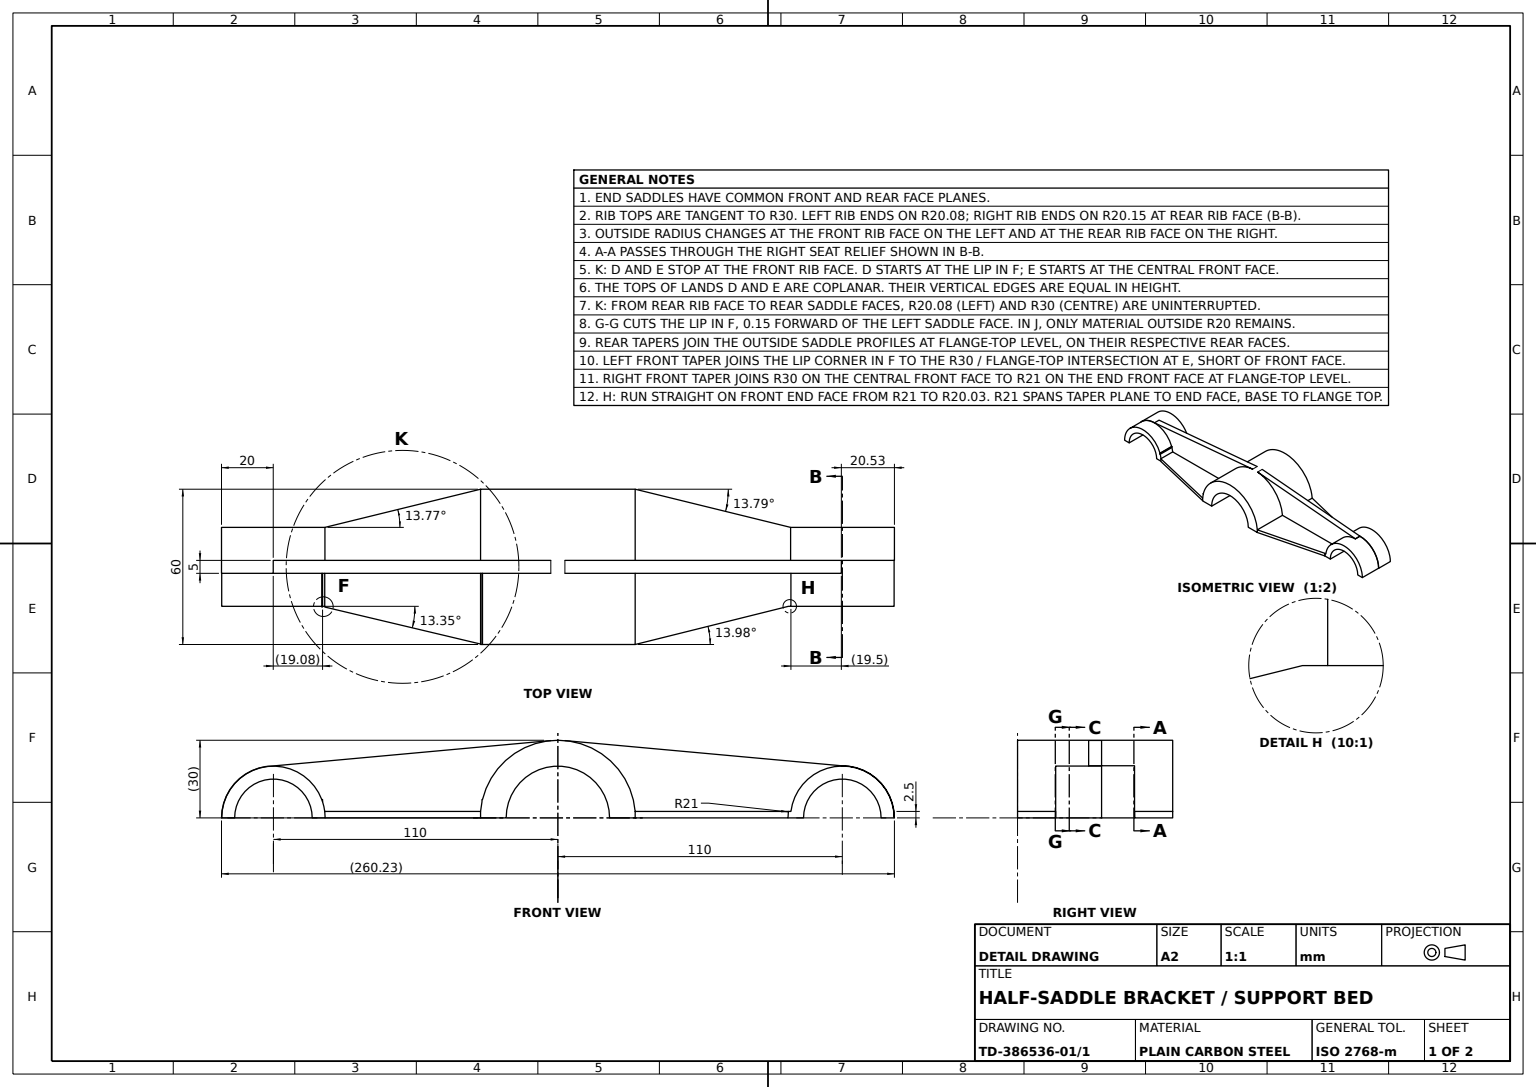
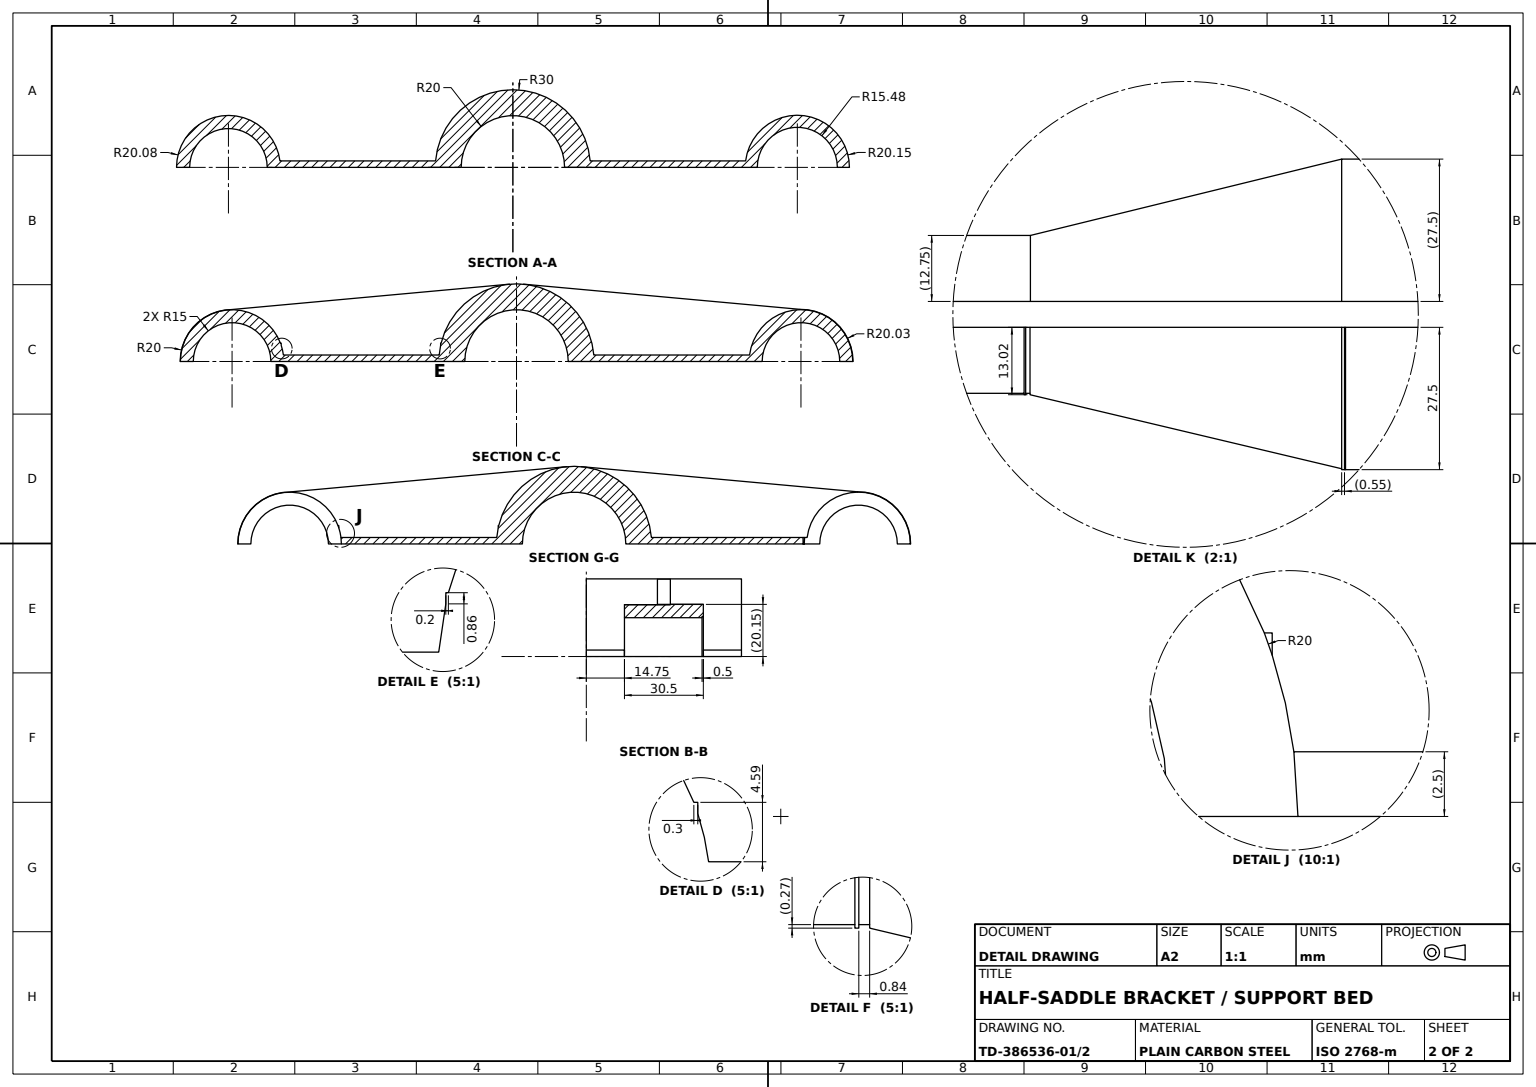
ISO-10303-21;
HEADER;
FILE_DESCRIPTION((''),'2;1');
FILE_NAME('','',(''),(''),'','','');
FILE_SCHEMA(('AUTOMOTIVE_DESIGN'));
ENDSEC;
DATA;
#1=APPLICATION_CONTEXT('');
#2=PRODUCT_CONTEXT('',#1,'mechanical');
#3=PRODUCT('','','',(#2));
#4=PRODUCT_DEFINITION_FORMATION('','',#3);
#5=PRODUCT_DEFINITION_CONTEXT('',#1,'design');
#6=PRODUCT_DEFINITION('','',#4,#5);
#7=PRODUCT_DEFINITION_SHAPE('','',#6);
#8=(LENGTH_UNIT()NAMED_UNIT(*)SI_UNIT(.MILLI.,.METRE.));
#9=(NAMED_UNIT(*)PLANE_ANGLE_UNIT()SI_UNIT($,.RADIAN.));
#10=(NAMED_UNIT(*)SI_UNIT($,.STERADIAN.)SOLID_ANGLE_UNIT());
#11=UNCERTAINTY_MEASURE_WITH_UNIT(LENGTH_MEASURE(1.E-05),#8,'distance_accuracy_value','');
#12=(GEOMETRIC_REPRESENTATION_CONTEXT(3)GLOBAL_UNCERTAINTY_ASSIGNED_CONTEXT((#11))GLOBAL_UNIT_ASSIGNED_CONTEXT((#8,#9,#10))REPRESENTATION_CONTEXT('',''));
#13=CARTESIAN_POINT('',(109.62431,20.147505,70.));
#14=VERTEX_POINT('',#13);
#15=CARTESIAN_POINT('',(109.62431,20.027015,70.));
#16=VERTEX_POINT('',#15);
#17=CARTESIAN_POINT('',(109.62431,0.,70.));
#18=DIRECTION('',(0.,-1.,0.));
#19=VECTOR('',#18,1000.);
#20=LINE('',#17,#19);
#21=EDGE_CURVE('',#14,#16,#20,.T.);
#22=ORIENTED_EDGE('',*,*,#21,.F.);
#23=CARTESIAN_POINT('',(109.62431,20.147505,75.));
#24=VERTEX_POINT('',#23);
#25=DIRECTION('',(0.,0.,1.));
#26=VECTOR('',#25,1000.);
#27=LINE('',#13,#26);
#28=EDGE_CURVE('',#14,#24,#27,.T.);
#29=ORIENTED_EDGE('',*,*,#28,.T.);
#30=CARTESIAN_POINT('',(109.62431,20.027015,75.));
#31=VERTEX_POINT('',#30);
#32=CARTESIAN_POINT('',(109.62431,0.,75.));
#33=LINE('',#32,#19);
#34=EDGE_CURVE('',#24,#31,#33,.T.);
#35=ORIENTED_EDGE('',*,*,#34,.T.);
#36=DIRECTION('',(0.,0.,-1.));
#37=VECTOR('',#36,1000.);
#38=LINE('',#30,#37);
#39=EDGE_CURVE('',#31,#16,#38,.T.);
#40=ORIENTED_EDGE('',*,*,#39,.T.);
#41=EDGE_LOOP('',(#22,#29,#35,#40));
#42=FACE_OUTER_BOUND('',#41,.T.);
#43=DIRECTION('',(-1.,0.,0.));
#44=AXIS2_PLACEMENT_3D('',#17,#43,#25);
#45=PLANE('',#44);
#46=ADVANCED_FACE('',(#42),#45,.F.);
#47=CARTESIAN_POINT('',(-89.923483,0.,57.211703));
#48=VERTEX_POINT('',#47);
#49=CARTESIAN_POINT('',(-29.895652,0.,42.5));
#50=VERTEX_POINT('',#49);
#51=CARTESIAN_POINT('',(-90.079745,0.,57.25));
#52=DIRECTION('',(0.97125614,0.,-0.238036784));
#53=VECTOR('',#52,1000.);
#54=LINE('',#51,#53);
#55=EDGE_CURVE('',#48,#50,#54,.T.);
#56=ORIENTED_EDGE('',*,*,#55,.F.);
#57=CARTESIAN_POINT('',(-90.079745,2.5,57.25));
#58=VERTEX_POINT('',#57);
#59=CARTESIAN_POINT('',(-89.923483,0.836045,57.211703));
#60=CARTESIAN_POINT('',(-89.975638,1.670462,57.224485));
#61=(BOUNDED_CURVE()B_SPLINE_CURVE(3,(#47,#59,#60,#57),.UNSPECIFIED.,.F.,.T.)B_SPLINE_CURVE_WITH_KNOTS((4,4),(0.,0.12484767),.UNSPECIFIED.)CURVE()GEOMETRIC_REPRESENTATION_ITEM()RATIONAL_B_SPLINE_CURVE((1.,0.99870151,0.99870151,1.))REPRESENTATION_ITEM(''));
#62=EDGE_CURVE('',#48,#58,#61,.T.);
#63=ORIENTED_EDGE('',*,*,#62,.T.);
#64=CARTESIAN_POINT('',(-29.895652,2.5,42.5));
#65=VERTEX_POINT('',#64);
#66=CARTESIAN_POINT('',(-1.693933,2.5,35.588284));
#67=DIRECTION('',(-0.97125614,0.,0.238036784));
#68=VECTOR('',#67,1000.);
#69=LINE('',#66,#68);
#70=EDGE_CURVE('',#65,#58,#69,.T.);
#71=ORIENTED_EDGE('',*,*,#70,.F.);
#72=CARTESIAN_POINT('',(-29.895652,68.5,42.5));
#73=LINE('',#72,#19);
#74=EDGE_CURVE('',#65,#50,#73,.T.);
#75=ORIENTED_EDGE('',*,*,#74,.T.);
#76=EDGE_LOOP('',(#56,#63,#71,#75));
#77=FACE_OUTER_BOUND('',#76,.T.);
#78=CARTESIAN_POINT('',(-90.079745,68.5,57.25));
#79=DIRECTION('',(-0.238036784,0.,-0.97125614));
#80=AXIS2_PLACEMENT_3D('',#78,#79,#67);
#81=PLANE('',#80);
#82=ADVANCED_FACE('',(#77),#81,.T.);
#83=CARTESIAN_POINT('',(29.895652,2.5,42.5));
#84=VERTEX_POINT('',#83);
#85=CARTESIAN_POINT('',(29.895652,2.5,70.));
#86=VERTEX_POINT('',#85);
#87=LINE('',#83,#26);
#88=EDGE_CURVE('',#84,#86,#87,.T.);
#89=ORIENTED_EDGE('',*,*,#88,.F.);
#90=CARTESIAN_POINT('',(0.,0.,42.5));
#91=AXIS2_PLACEMENT_3D('',#90,#36,#43);
#92=CIRCLE('',#91,30.);
#93=EDGE_CURVE('',#65,#84,#92,.T.);
#94=ORIENTED_EDGE('',*,*,#93,.F.);
#95=CARTESIAN_POINT('',(-29.895652,2.5,70.));
#96=VERTEX_POINT('',#95);
#97=LINE('',#64,#26);
#98=EDGE_CURVE('',#65,#96,#97,.T.);
#99=ORIENTED_EDGE('',*,*,#98,.T.);
#100=CARTESIAN_POINT('',(-2.727273,29.875776,70.));
#101=VERTEX_POINT('',#100);
#102=CARTESIAN_POINT('',(0.,0.,70.));
#103=AXIS2_PLACEMENT_3D('',#102,#25,#43);
#104=CIRCLE('',#103,30.);
#105=EDGE_CURVE('',#101,#96,#104,.T.);
#106=ORIENTED_EDGE('',*,*,#105,.F.);
#107=CARTESIAN_POINT('',(-2.727273,29.875776,75.));
#108=VERTEX_POINT('',#107);
#109=LINE('',#107,#37);
#110=EDGE_CURVE('',#108,#101,#109,.T.);
#111=ORIENTED_EDGE('',*,*,#110,.F.);
#112=CARTESIAN_POINT('',(-29.149589,7.092351,75.));
#113=VERTEX_POINT('',#112);
#114=CARTESIAN_POINT('',(0.,0.,75.));
#115=DIRECTION('',(1.,0.,0.));
#116=AXIS2_PLACEMENT_3D('',#114,#25,#115);
#117=CIRCLE('',#116,30.);
#118=EDGE_CURVE('',#108,#113,#117,.T.);
#119=ORIENTED_EDGE('',*,*,#118,.T.);
#120=CARTESIAN_POINT('',(-29.149589,7.092351,102.5));
#121=VERTEX_POINT('',#120);
#122=LINE('',#120,#37);
#123=EDGE_CURVE('',#121,#113,#122,.T.);
#124=ORIENTED_EDGE('',*,*,#123,.F.);
#125=CARTESIAN_POINT('',(29.895652,2.5,102.5));
#126=VERTEX_POINT('',#125);
#127=CARTESIAN_POINT('',(0.,0.,102.5));
#128=AXIS2_PLACEMENT_3D('',#127,#25,#115);
#129=CIRCLE('',#128,30.);
#130=EDGE_CURVE('',#126,#121,#129,.T.);
#131=ORIENTED_EDGE('',*,*,#130,.F.);
#132=CARTESIAN_POINT('',(29.895652,2.5,75.));
#133=VERTEX_POINT('',#132);
#134=LINE('',#125,#37);
#135=EDGE_CURVE('',#126,#133,#134,.T.);
#136=ORIENTED_EDGE('',*,*,#135,.T.);
#137=CARTESIAN_POINT('',(2.718944,29.876535,75.));
#138=VERTEX_POINT('',#137);
#139=EDGE_CURVE('',#133,#138,#117,.T.);
#140=ORIENTED_EDGE('',*,*,#139,.T.);
#141=CARTESIAN_POINT('',(2.718944,29.876535,70.));
#142=VERTEX_POINT('',#141);
#143=LINE('',#141,#26);
#144=EDGE_CURVE('',#142,#138,#143,.T.);
#145=ORIENTED_EDGE('',*,*,#144,.F.);
#146=EDGE_CURVE('',#86,#142,#104,.T.);
#147=ORIENTED_EDGE('',*,*,#146,.F.);
#148=EDGE_LOOP('',(#89,#94,#99,#106,#111,#119,#124,#131,#136,#140,#145,#147));
#149=FACE_OUTER_BOUND('',#148,.T.);
#150=CARTESIAN_POINT('',(0.,0.,20.));
#151=AXIS2_PLACEMENT_3D('',#150,#36,#43);
#152=CYLINDRICAL_SURFACE('',#151,30.);
#153=ADVANCED_FACE('',(#149),#152,.T.);
#154=CARTESIAN_POINT('',(-90.156865,2.5,88.021244));
#155=VERTEX_POINT('',#154);
#156=CARTESIAN_POINT('',(-90.,0.,88.058473));
#157=VERTEX_POINT('',#156);
#158=CARTESIAN_POINT('',(-90.052357,1.670491,88.046047));
#159=CARTESIAN_POINT('',(-90.,0.836066,88.058473));
#160=(BOUNDED_CURVE()B_SPLINE_CURVE(3,(#154,#158,#159,#156),.UNSPECIFIED.,.F.,.F.)B_SPLINE_CURVE_WITH_KNOTS((4,4),(6.157857476,6.283185307),.UNSPECIFIED.)CURVE()GEOMETRIC_REPRESENTATION_ITEM()RATIONAL_B_SPLINE_CURVE((1.,0.998691506,0.998691506,1.))REPRESENTATION_ITEM(''));
#161=EDGE_CURVE('',#155,#157,#160,.T.);
#162=ORIENTED_EDGE('',*,*,#161,.F.);
#163=CARTESIAN_POINT('',(-90.156865,2.5,87.75));
#164=VERTEX_POINT('',#163);
#165=CARTESIAN_POINT('',(-90.156865,2.5,102.5));
#166=LINE('',#165,#37);
#167=EDGE_CURVE('',#155,#164,#166,.T.);
#168=ORIENTED_EDGE('',*,*,#167,.T.);
#169=CARTESIAN_POINT('',(-90.,0.,87.75));
#170=VERTEX_POINT('',#169);
#171=CARTESIAN_POINT('',(-110.,0.,87.75));
#172=AXIS2_PLACEMENT_3D('',#171,#25,#115);
#173=CIRCLE('',#172,20.);
#174=EDGE_CURVE('',#170,#164,#173,.T.);
#175=ORIENTED_EDGE('',*,*,#174,.F.);
#176=LINE('',#169,#26);
#177=EDGE_CURVE('',#170,#157,#176,.T.);
#178=ORIENTED_EDGE('',*,*,#177,.T.);
#179=EDGE_LOOP('',(#162,#168,#175,#178));
#180=FACE_OUTER_BOUND('',#179,.T.);
#181=CYLINDRICAL_SURFACE('',#172,20.);
#182=ADVANCED_FACE('',(#180),#181,.F.);
#183=CARTESIAN_POINT('',(-91.299771,7.092351,75.));
#184=VERTEX_POINT('',#183);
#185=CARTESIAN_POINT('',(-130.,0.,75.));
#186=VERTEX_POINT('',#185);
#187=CARTESIAN_POINT('',(-110.,0.,75.));
#188=AXIS2_PLACEMENT_3D('',#187,#25,#43);
#189=CIRCLE('',#188,20.);
#190=EDGE_CURVE('',#184,#186,#189,.T.);
#191=ORIENTED_EDGE('',*,*,#190,.T.);
#192=CARTESIAN_POINT('',(-130.,0.,87.75));
#193=VERTEX_POINT('',#192);
#194=CARTESIAN_POINT('',(-130.,0.,102.5));
#195=LINE('',#194,#26);
#196=EDGE_CURVE('',#186,#193,#195,.T.);
#197=ORIENTED_EDGE('',*,*,#196,.T.);
#198=CARTESIAN_POINT('',(-91.299771,7.092351,87.75));
#199=VERTEX_POINT('',#198);
#200=EDGE_CURVE('',#199,#193,#173,.T.);
#201=ORIENTED_EDGE('',*,*,#200,.F.);
#202=CARTESIAN_POINT('',(-91.299771,7.092351,102.5));
#203=LINE('',#202,#37);
#204=EDGE_CURVE('',#199,#184,#203,.T.);
#205=ORIENTED_EDGE('',*,*,#204,.T.);
#206=EDGE_LOOP('',(#191,#197,#201,#205));
#207=FACE_OUTER_BOUND('',#206,.T.);
#208=CARTESIAN_POINT('',(-110.,0.,102.5));
#209=AXIS2_PLACEMENT_3D('',#208,#36,#43);
#210=CYLINDRICAL_SURFACE('',#209,20.);
#211=ADVANCED_FACE('',(#207),#210,.T.);
#212=CARTESIAN_POINT('',(29.895652,0.,102.5));
#213=VERTEX_POINT('',#212);
#214=CARTESIAN_POINT('',(29.895652,-99.5,102.5));
#215=DIRECTION('',(0.,1.,0.));
#216=VECTOR('',#215,1000.);
#217=LINE('',#214,#216);
#218=EDGE_CURVE('',#213,#126,#217,.T.);
#219=ORIENTED_EDGE('',*,*,#218,.F.);
#220=CARTESIAN_POINT('',(89.,0.,87.787175));
#221=VERTEX_POINT('',#220);
#222=DIRECTION('',(-0.970386397,0.,0.241557946));
#223=VECTOR('',#222,1000.);
#224=LINE('',#212,#223);
#225=EDGE_CURVE('',#221,#213,#224,.T.);
#226=ORIENTED_EDGE('',*,*,#225,.F.);
#227=CARTESIAN_POINT('',(89.149341,2.5,87.75));
#228=VERTEX_POINT('',#227);
#229=CARTESIAN_POINT('',(89.049839,1.670133,87.774769));
#230=CARTESIAN_POINT('',(89.,0.83581,87.787175));
#231=(BOUNDED_CURVE()B_SPLINE_CURVE(3,(#227,#229,#230,#220),.UNSPECIFIED.,.F.,.F.)B_SPLINE_CURVE_WITH_KNOTS((4,4),(3.022262029,3.141592654),.UNSPECIFIED.)CURVE()GEOMETRIC_REPRESENTATION_ITEM()RATIONAL_B_SPLINE_CURVE((1.,0.998813702,0.998813702,1.))REPRESENTATION_ITEM(''));
#232=EDGE_CURVE('',#228,#221,#231,.T.);
#233=ORIENTED_EDGE('',*,*,#232,.F.);
#234=CARTESIAN_POINT('',(1.744419,2.5,109.507677));
#235=DIRECTION('',(0.970386397,0.,-0.241557946));
#236=VECTOR('',#235,1000.);
#237=LINE('',#234,#236);
#238=EDGE_CURVE('',#126,#228,#237,.T.);
#239=ORIENTED_EDGE('',*,*,#238,.F.);
#240=EDGE_LOOP('',(#219,#226,#233,#239));
#241=FACE_OUTER_BOUND('',#240,.T.);
#242=DIRECTION('',(0.241557946,0.,0.970386397));
#243=AXIS2_PLACEMENT_3D('',#214,#242,#235);
#244=PLANE('',#243);
#245=ADVANCED_FACE('',(#241),#244,.T.);
#246=CARTESIAN_POINT('',(-110.074279,20.07638,70.));
#247=VERTEX_POINT('',#246);
#248=CARTESIAN_POINT('',(-90.079745,2.5,70.));
#249=VERTEX_POINT('',#248);
#250=CARTESIAN_POINT('',(-110.,0.,70.));
#251=AXIS2_PLACEMENT_3D('',#250,#36,#43);
#252=CIRCLE('',#251,20.076517);
#253=EDGE_CURVE('',#247,#249,#252,.T.);
#254=ORIENTED_EDGE('',*,*,#253,.F.);
#255=DIRECTION('',(-0.995859195,-0.090909091,0.));
#256=VECTOR('',#255,1000.);
#257=LINE('',#100,#256);
#258=EDGE_CURVE('',#101,#247,#257,.T.);
#259=ORIENTED_EDGE('',*,*,#258,.F.);
#260=ORIENTED_EDGE('',*,*,#105,.T.);
#261=CARTESIAN_POINT('',(0.,2.5,70.));
#262=VECTOR('',#43,1000.);
#263=LINE('',#261,#262);
#264=EDGE_CURVE('',#96,#249,#263,.T.);
#265=ORIENTED_EDGE('',*,*,#264,.T.);
#266=EDGE_LOOP('',(#254,#259,#260,#265));
#267=FACE_OUTER_BOUND('',#266,.T.);
#268=AXIS2_PLACEMENT_3D('',#102,#36,#43);
#269=PLANE('',#268);
#270=ADVANCED_FACE('',(#267),#269,.T.);
#271=CARTESIAN_POINT('',(-90.156865,2.5,75.));
#272=VERTEX_POINT('',#271);
#273=EDGE_CURVE('',#164,#272,#166,.T.);
#274=ORIENTED_EDGE('',*,*,#273,.T.);
#275=CARTESIAN_POINT('',(-90.995037,6.229877,75.));
#276=VERTEX_POINT('',#275);
#277=EDGE_CURVE('',#272,#276,#189,.T.);
#278=ORIENTED_EDGE('',*,*,#277,.T.);
#279=CARTESIAN_POINT('',(-90.995037,6.229877,87.75));
#280=VERTEX_POINT('',#279);
#281=CARTESIAN_POINT('',(-90.995037,6.229877,102.5));
#282=LINE('',#281,#37);
#283=EDGE_CURVE('',#280,#276,#282,.T.);
#284=ORIENTED_EDGE('',*,*,#283,.F.);
#285=EDGE_CURVE('',#164,#280,#173,.T.);
#286=ORIENTED_EDGE('',*,*,#285,.F.);
#287=EDGE_LOOP('',(#274,#278,#284,#286));
#288=FACE_OUTER_BOUND('',#287,.T.);
#289=ADVANCED_FACE('',(#288),#210,.T.);
#290=CARTESIAN_POINT('',(-90.995037,7.092351,75.));
#291=VERTEX_POINT('',#290);
#292=CARTESIAN_POINT('',(-90.995037,0.,75.));
#293=LINE('',#292,#19);
#294=EDGE_CURVE('',#291,#276,#293,.T.);
#295=ORIENTED_EDGE('',*,*,#294,.F.);
#296=CARTESIAN_POINT('',(-90.995037,7.092351,88.021244));
#297=VERTEX_POINT('',#296);
#298=CARTESIAN_POINT('',(-90.995037,7.092351,102.5));
#299=LINE('',#298,#37);
#300=EDGE_CURVE('',#297,#291,#299,.T.);
#301=ORIENTED_EDGE('',*,*,#300,.F.);
#302=CARTESIAN_POINT('',(-90.995037,6.229877,88.021244));
#303=VERTEX_POINT('',#302);
#304=CARTESIAN_POINT('',(-90.995037,-57.229877,88.021244));
#305=LINE('',#304,#216);
#306=EDGE_CURVE('',#303,#297,#305,.T.);
#307=ORIENTED_EDGE('',*,*,#306,.F.);
#308=EDGE_CURVE('',#303,#280,#282,.T.);
#309=ORIENTED_EDGE('',*,*,#308,.T.);
#310=ORIENTED_EDGE('',*,*,#283,.T.);
#311=EDGE_LOOP('',(#295,#301,#307,#309,#310));
#312=FACE_OUTER_BOUND('',#311,.T.);
#313=CARTESIAN_POINT('',(-90.995037,-57.229877,75.));
#314=AXIS2_PLACEMENT_3D('',#313,#115,#36);
#315=PLANE('',#314);
#316=ADVANCED_FACE('',(#312),#315,.T.);
#317=CARTESIAN_POINT('',(125.480421,0.,57.75));
#318=VERTEX_POINT('',#317);
#319=CARTESIAN_POINT('',(94.519579,0.,57.75));
#320=VERTEX_POINT('',#319);
#321=CARTESIAN_POINT('',(110.,0.,57.75));
#322=AXIS2_PLACEMENT_3D('',#321,#25,#115);
#323=CIRCLE('',#322,15.480421);
#324=EDGE_CURVE('',#318,#320,#323,.T.);
#325=ORIENTED_EDGE('',*,*,#324,.T.);
#326=CARTESIAN_POINT('',(94.519579,0.,57.25));
#327=VERTEX_POINT('',#326);
#328=CARTESIAN_POINT('',(94.519579,0.,47.75));
#329=LINE('',#328,#37);
#330=EDGE_CURVE('',#320,#327,#329,.T.);
#331=ORIENTED_EDGE('',*,*,#330,.T.);
#332=CARTESIAN_POINT('',(125.480421,0.,57.25));
#333=VERTEX_POINT('',#332);
#334=CARTESIAN_POINT('',(110.,0.,57.25));
#335=AXIS2_PLACEMENT_3D('',#334,#36,#43);
#336=CIRCLE('',#335,15.480421);
#337=EDGE_CURVE('',#327,#333,#336,.T.);
#338=ORIENTED_EDGE('',*,*,#337,.T.);
#339=CARTESIAN_POINT('',(125.480421,0.,47.75));
#340=LINE('',#339,#26);
#341=EDGE_CURVE('',#333,#318,#340,.T.);
#342=ORIENTED_EDGE('',*,*,#341,.T.);
#343=EDGE_LOOP('',(#325,#331,#338,#342));
#344=FACE_OUTER_BOUND('',#343,.T.);
#345=CARTESIAN_POINT('',(110.,0.,47.75));
#346=AXIS2_PLACEMENT_3D('',#345,#25,#115);
#347=CYLINDRICAL_SURFACE('',#346,15.480421);
#348=ADVANCED_FACE('',(#344),#347,.F.);
#349=CARTESIAN_POINT('',(-91.299771,7.092351,88.021244));
#350=VERTEX_POINT('',#349);
#351=EDGE_CURVE('',#350,#199,#203,.T.);
#352=ORIENTED_EDGE('',*,*,#351,.T.);
#353=EDGE_CURVE('',#280,#199,#173,.T.);
#354=ORIENTED_EDGE('',*,*,#353,.F.);
#355=ORIENTED_EDGE('',*,*,#308,.F.);
#356=CARTESIAN_POINT('',(-110.,0.,88.021244));
#357=AXIS2_PLACEMENT_3D('',#356,#25,#43);
#358=CIRCLE('',#357,20.);
#359=EDGE_CURVE('',#303,#350,#358,.T.);
#360=ORIENTED_EDGE('',*,*,#359,.T.);
#361=EDGE_LOOP('',(#352,#354,#355,#360));
#362=FACE_OUTER_BOUND('',#361,.T.);
#363=ADVANCED_FACE('',(#362),#181,.F.);
#364=CARTESIAN_POINT('',(130.151008,0.,70.));
#365=VERTEX_POINT('',#364);
#366=CARTESIAN_POINT('',(110.,0.,70.));
#367=AXIS2_PLACEMENT_3D('',#366,#36,#43);
#368=CIRCLE('',#367,20.151008);
#369=EDGE_CURVE('',#14,#365,#368,.T.);
#370=ORIENTED_EDGE('',*,*,#369,.T.);
#371=CARTESIAN_POINT('',(130.151008,0.,57.25));
#372=VERTEX_POINT('',#371);
#373=CARTESIAN_POINT('',(130.151008,0.,42.5));
#374=LINE('',#373,#37);
#375=EDGE_CURVE('',#365,#372,#374,.T.);
#376=ORIENTED_EDGE('',*,*,#375,.T.);
#377=CARTESIAN_POINT('',(90.004673,2.5,57.25));
#378=VERTEX_POINT('',#377);
#379=CIRCLE('',#335,20.151008);
#380=EDGE_CURVE('',#378,#372,#379,.T.);
#381=ORIENTED_EDGE('',*,*,#380,.F.);
#382=CARTESIAN_POINT('',(90.004673,2.5,70.));
#383=VERTEX_POINT('',#382);
#384=CARTESIAN_POINT('',(90.004673,2.5,42.5));
#385=LINE('',#384,#26);
#386=EDGE_CURVE('',#378,#383,#385,.T.);
#387=ORIENTED_EDGE('',*,*,#386,.T.);
#388=AXIS2_PLACEMENT_3D('',#366,#36,#115);
#389=CIRCLE('',#388,20.151008);
#390=EDGE_CURVE('',#383,#14,#389,.T.);
#391=ORIENTED_EDGE('',*,*,#390,.T.);
#392=EDGE_LOOP('',(#370,#376,#381,#387,#391));
#393=FACE_OUTER_BOUND('',#392,.T.);
#394=CARTESIAN_POINT('',(110.,0.,42.5));
#395=AXIS2_PLACEMENT_3D('',#394,#25,#115);
#396=CYLINDRICAL_SURFACE('',#395,20.151008);
#397=ADVANCED_FACE('',(#393),#396,.T.);
#398=CARTESIAN_POINT('',(20.,0.,102.5));
#399=VERTEX_POINT('',#398);
#400=CARTESIAN_POINT('',(-20.,0.,102.5));
#401=VERTEX_POINT('',#400);
#402=CIRCLE('',#128,20.);
#403=EDGE_CURVE('',#399,#401,#402,.T.);
#404=ORIENTED_EDGE('',*,*,#403,.T.);
#405=CARTESIAN_POINT('',(-20.,0.,42.5));
#406=VERTEX_POINT('',#405);
#407=CARTESIAN_POINT('',(-20.,0.,92.5));
#408=LINE('',#407,#37);
#409=EDGE_CURVE('',#401,#406,#408,.T.);
#410=ORIENTED_EDGE('',*,*,#409,.T.);
#411=CARTESIAN_POINT('',(20.,0.,42.5));
#412=VERTEX_POINT('',#411);
#413=AXIS2_PLACEMENT_3D('',#90,#25,#115);
#414=CIRCLE('',#413,20.);
#415=EDGE_CURVE('',#412,#406,#414,.T.);
#416=ORIENTED_EDGE('',*,*,#415,.F.);
#417=CARTESIAN_POINT('',(20.,0.,92.5));
#418=LINE('',#417,#26);
#419=EDGE_CURVE('',#412,#399,#418,.T.);
#420=ORIENTED_EDGE('',*,*,#419,.T.);
#421=EDGE_LOOP('',(#404,#410,#416,#420));
#422=FACE_OUTER_BOUND('',#421,.T.);
#423=CARTESIAN_POINT('',(0.,0.,92.5));
#424=AXIS2_PLACEMENT_3D('',#423,#25,#115);
#425=CYLINDRICAL_SURFACE('',#424,20.);
#426=ADVANCED_FACE('',(#422),#425,.F.);
#427=CARTESIAN_POINT('',(-29.346016,6.229877,102.5));
#428=VERTEX_POINT('',#427);
#429=CARTESIAN_POINT('',(-29.346016,7.092351,102.5));
#430=VERTEX_POINT('',#429);
#431=CARTESIAN_POINT('',(-29.346016,-57.229877,102.5));
#432=LINE('',#431,#216);
#433=EDGE_CURVE('',#428,#430,#432,.T.);
#434=ORIENTED_EDGE('',*,*,#433,.T.);
#435=CARTESIAN_POINT('',(-29.346016,7.092351,75.));
#436=VERTEX_POINT('',#435);
#437=CARTESIAN_POINT('',(-29.346016,7.092351,176.5));
#438=LINE('',#437,#37);
#439=EDGE_CURVE('',#430,#436,#438,.T.);
#440=ORIENTED_EDGE('',*,*,#439,.T.);
#441=CARTESIAN_POINT('',(-29.346016,6.229877,75.));
#442=VERTEX_POINT('',#441);
#443=CARTESIAN_POINT('',(-29.346016,0.,75.));
#444=LINE('',#443,#19);
#445=EDGE_CURVE('',#436,#442,#444,.T.);
#446=ORIENTED_EDGE('',*,*,#445,.T.);
#447=CARTESIAN_POINT('',(-29.346016,6.229877,176.5));
#448=LINE('',#447,#37);
#449=EDGE_CURVE('',#428,#442,#448,.T.);
#450=ORIENTED_EDGE('',*,*,#449,.F.);
#451=EDGE_LOOP('',(#434,#440,#446,#450));
#452=FACE_OUTER_BOUND('',#451,.T.);
#453=CARTESIAN_POINT('',(-29.346016,0.,176.5));
#454=AXIS2_PLACEMENT_3D('',#453,#115,#36);
#455=PLANE('',#454);
#456=ADVANCED_FACE('',(#452),#455,.F.);
#457=CARTESIAN_POINT('',(-29.895652,2.5,102.5));
#458=VERTEX_POINT('',#457);
#459=CARTESIAN_POINT('',(-29.895652,2.5,102.322938));
#460=VERTEX_POINT('',#459);
#461=LINE('',#457,#37);
#462=EDGE_CURVE('',#458,#460,#461,.T.);
#463=ORIENTED_EDGE('',*,*,#462,.F.);
#464=EDGE_CURVE('',#428,#458,#129,.T.);
#465=ORIENTED_EDGE('',*,*,#464,.F.);
#466=ORIENTED_EDGE('',*,*,#449,.T.);
#467=CARTESIAN_POINT('',(-29.895652,2.5,75.));
#468=VERTEX_POINT('',#467);
#469=EDGE_CURVE('',#442,#468,#117,.T.);
#470=ORIENTED_EDGE('',*,*,#469,.T.);
#471=EDGE_CURVE('',#460,#468,#461,.T.);
#472=ORIENTED_EDGE('',*,*,#471,.F.);
#473=EDGE_LOOP('',(#463,#465,#466,#470,#472));
#474=FACE_OUTER_BOUND('',#473,.T.);
#475=ADVANCED_FACE('',(#474),#152,.T.);
#476=ORIENTED_EDGE('',*,*,#351,.F.);
#477=LINE('',#349,#262);
#478=EDGE_CURVE('',#297,#350,#477,.T.);
#479=ORIENTED_EDGE('',*,*,#478,.F.);
#480=ORIENTED_EDGE('',*,*,#300,.T.);
#481=VECTOR('',#115,1000.);
#482=LINE('',#183,#481);
#483=EDGE_CURVE('',#184,#291,#482,.T.);
#484=ORIENTED_EDGE('',*,*,#483,.F.);
#485=ORIENTED_EDGE('',*,*,#204,.F.);
#486=EDGE_LOOP('',(#476,#479,#480,#484,#485));
#487=FACE_OUTER_BOUND('',#486,.T.);
#488=AXIS2_PLACEMENT_3D('',#202,#215,#25);
#489=PLANE('',#488);
#490=ADVANCED_FACE('',(#487),#489,.T.);
#491=CARTESIAN_POINT('',(-29.895652,0.,102.322938));
#492=VERTEX_POINT('',#491);
#493=CARTESIAN_POINT('',(-29.895652,-78.5,102.322938));
#494=LINE('',#493,#216);
#495=EDGE_CURVE('',#492,#460,#494,.T.);
#496=ORIENTED_EDGE('',*,*,#495,.T.);
#497=CARTESIAN_POINT('',(-1.554298,2.5,109.049145));
#498=DIRECTION('',(0.972974086,0.,0.230914332));
#499=VECTOR('',#498,1000.);
#500=LINE('',#497,#499);
#501=EDGE_CURVE('',#155,#460,#500,.T.);
#502=ORIENTED_EDGE('',*,*,#501,.F.);
#503=ORIENTED_EDGE('',*,*,#161,.T.);
#504=CARTESIAN_POINT('',(-24.583348,0.,103.583698));
#505=DIRECTION('',(-0.972974086,0.,-0.230914332));
#506=VECTOR('',#505,1000.);
#507=LINE('',#504,#506);
#508=EDGE_CURVE('',#492,#157,#507,.T.);
#509=ORIENTED_EDGE('',*,*,#508,.F.);
#510=EDGE_LOOP('',(#496,#502,#503,#509));
#511=FACE_OUTER_BOUND('',#510,.T.);
#512=CARTESIAN_POINT('',(-24.583348,-78.5,103.583698));
#513=DIRECTION('',(-0.230914332,0.,0.972974086));
#514=AXIS2_PLACEMENT_3D('',#512,#513,#498);
#515=PLANE('',#514);
#516=ADVANCED_FACE('',(#511),#515,.T.);
#517=CARTESIAN_POINT('',(-110.074279,20.07638,75.));
#518=VERTEX_POINT('',#517);
#519=LINE('',#517,#37);
#520=EDGE_CURVE('',#518,#247,#519,.T.);
#521=ORIENTED_EDGE('',*,*,#520,.T.);
#522=ORIENTED_EDGE('',*,*,#253,.T.);
#523=CARTESIAN_POINT('',(-90.079745,2.5,42.5));
#524=LINE('',#523,#26);
#525=EDGE_CURVE('',#58,#249,#524,.T.);
#526=ORIENTED_EDGE('',*,*,#525,.F.);
#527=CARTESIAN_POINT('',(-130.076517,0.,57.25));
#528=VERTEX_POINT('',#527);
#529=CARTESIAN_POINT('',(-110.,0.,57.25));
#530=AXIS2_PLACEMENT_3D('',#529,#36,#43);
#531=CIRCLE('',#530,20.076517);
#532=EDGE_CURVE('',#528,#58,#531,.T.);
#533=ORIENTED_EDGE('',*,*,#532,.F.);
#534=CARTESIAN_POINT('',(-130.076517,0.,75.));
#535=VERTEX_POINT('',#534);
#536=LINE('',#534,#37);
#537=EDGE_CURVE('',#535,#528,#536,.T.);
#538=ORIENTED_EDGE('',*,*,#537,.F.);
#539=AXIS2_PLACEMENT_3D('',#187,#36,#43);
#540=CIRCLE('',#539,20.076517);
#541=EDGE_CURVE('',#535,#518,#540,.T.);
#542=ORIENTED_EDGE('',*,*,#541,.T.);
#543=EDGE_LOOP('',(#521,#522,#526,#533,#538,#542));
#544=FACE_OUTER_BOUND('',#543,.T.);
#545=CYLINDRICAL_SURFACE('',#539,20.076517);
#546=ADVANCED_FACE('',(#544),#545,.T.);
#547=ORIENTED_EDGE('',*,*,#174,.T.);
#548=ORIENTED_EDGE('',*,*,#285,.T.);
#549=ORIENTED_EDGE('',*,*,#353,.T.);
#550=ORIENTED_EDGE('',*,*,#200,.T.);
#551=CARTESIAN_POINT('',(-125.,0.,87.75));
#552=VERTEX_POINT('',#551);
#553=LINE('',#171,#262);
#554=EDGE_CURVE('',#552,#193,#553,.T.);
#555=ORIENTED_EDGE('',*,*,#554,.F.);
#556=CARTESIAN_POINT('',(-95.,0.,87.75));
#557=VERTEX_POINT('',#556);
#558=AXIS2_PLACEMENT_3D('',#171,#36,#115);
#559=CIRCLE('',#558,15.);
#560=EDGE_CURVE('',#552,#557,#559,.T.);
#561=ORIENTED_EDGE('',*,*,#560,.T.);
#562=EDGE_CURVE('',#170,#557,#553,.T.);
#563=ORIENTED_EDGE('',*,*,#562,.F.);
#564=EDGE_LOOP('',(#547,#548,#549,#550,#555,#561,#563));
#565=FACE_OUTER_BOUND('',#564,.T.);
#566=PLANE('',#172);
#567=ADVANCED_FACE('',(#565),#566,.T.);
#568=CARTESIAN_POINT('',(130.030539,0.,70.));
#569=VERTEX_POINT('',#568);
#570=LINE('',#366,#481);
#571=EDGE_CURVE('',#569,#365,#570,.T.);
#572=ORIENTED_EDGE('',*,*,#571,.F.);
#573=CARTESIAN_POINT('',(130.030539,0.,87.75));
#574=VERTEX_POINT('',#573);
#575=CARTESIAN_POINT('',(130.030539,0.,75.));
#576=LINE('',#575,#26);
#577=EDGE_CURVE('',#569,#574,#576,.T.);
#578=ORIENTED_EDGE('',*,*,#577,.T.);
#579=CARTESIAN_POINT('',(125.,0.,87.75));
#580=VERTEX_POINT('',#579);
#581=CARTESIAN_POINT('',(110.,0.,87.75));
#582=LINE('',#581,#262);
#583=EDGE_CURVE('',#574,#580,#582,.T.);
#584=ORIENTED_EDGE('',*,*,#583,.T.);
#585=CARTESIAN_POINT('',(125.,0.,57.75));
#586=VERTEX_POINT('',#585);
#587=CARTESIAN_POINT('',(125.,0.,77.75));
#588=LINE('',#587,#26);
#589=EDGE_CURVE('',#586,#580,#588,.T.);
#590=ORIENTED_EDGE('',*,*,#589,.F.);
#591=LINE('',#321,#262);
#592=EDGE_CURVE('',#318,#586,#591,.T.);
#593=ORIENTED_EDGE('',*,*,#592,.F.);
#594=ORIENTED_EDGE('',*,*,#341,.F.);
#595=LINE('',#334,#481);
#596=EDGE_CURVE('',#333,#372,#595,.T.);
#597=ORIENTED_EDGE('',*,*,#596,.T.);
#598=ORIENTED_EDGE('',*,*,#375,.F.);
#599=EDGE_LOOP('',(#572,#578,#584,#590,#593,#594,#597,#598));
#600=FACE_OUTER_BOUND('',#599,.T.);
#601=CARTESIAN_POINT('',(0.,0.,-144.));
#602=AXIS2_PLACEMENT_3D('',#601,#215,#25);
#603=PLANE('',#602);
#604=ADVANCED_FACE('',(#600),#603,.F.);
#605=ORIENTED_EDGE('',*,*,#415,.T.);
#606=LINE('',#90,#481);
#607=EDGE_CURVE('',#50,#406,#606,.T.);
#608=ORIENTED_EDGE('',*,*,#607,.F.);
#609=ORIENTED_EDGE('',*,*,#74,.F.);
#610=ORIENTED_EDGE('',*,*,#93,.T.);
#611=CARTESIAN_POINT('',(29.895652,0.,42.5));
#612=VERTEX_POINT('',#611);
#613=CARTESIAN_POINT('',(29.895652,-57.5,42.5));
#614=LINE('',#613,#216);
#615=EDGE_CURVE('',#612,#84,#614,.T.);
#616=ORIENTED_EDGE('',*,*,#615,.F.);
#617=EDGE_CURVE('',#412,#612,#606,.T.);
#618=ORIENTED_EDGE('',*,*,#617,.F.);
#619=EDGE_LOOP('',(#605,#608,#609,#610,#616,#618));
#620=FACE_OUTER_BOUND('',#619,.T.);
#621=PLANE('',#91);
#622=ADVANCED_FACE('',(#620),#621,.T.);
#623=CARTESIAN_POINT('',(95.,0.,57.75));
#624=VERTEX_POINT('',#623);
#625=CIRCLE('',#322,15.);
#626=EDGE_CURVE('',#586,#624,#625,.T.);
#627=ORIENTED_EDGE('',*,*,#626,.T.);
#628=EDGE_CURVE('',#624,#320,#591,.T.);
#629=ORIENTED_EDGE('',*,*,#628,.T.);
#630=ORIENTED_EDGE('',*,*,#324,.F.);
#631=ORIENTED_EDGE('',*,*,#592,.T.);
#632=EDGE_LOOP('',(#627,#629,#630,#631));
#633=FACE_OUTER_BOUND('',#632,.T.);
#634=PLANE('',#322);
#635=ADVANCED_FACE('',(#633),#634,.F.);
#636=ORIENTED_EDGE('',*,*,#471,.T.);
#637=CARTESIAN_POINT('',(0.,2.5,75.));
#638=LINE('',#637,#481);
#639=EDGE_CURVE('',#272,#468,#638,.T.);
#640=ORIENTED_EDGE('',*,*,#639,.F.);
#641=ORIENTED_EDGE('',*,*,#273,.F.);
#642=ORIENTED_EDGE('',*,*,#167,.F.);
#643=ORIENTED_EDGE('',*,*,#501,.T.);
#644=EDGE_LOOP('',(#636,#640,#641,#642,#643));
#645=FACE_OUTER_BOUND('',#644,.T.);
#646=CARTESIAN_POINT('',(0.,2.5,102.5));
#647=AXIS2_PLACEMENT_3D('',#646,#215,#43);
#648=PLANE('',#647);
#649=ADVANCED_FACE('',(#645),#648,.T.);
#650=LINE('',#107,#256);
#651=EDGE_CURVE('',#108,#518,#650,.T.);
#652=ORIENTED_EDGE('',*,*,#651,.F.);
#653=ORIENTED_EDGE('',*,*,#110,.T.);
#654=ORIENTED_EDGE('',*,*,#258,.T.);
#655=ORIENTED_EDGE('',*,*,#520,.F.);
#656=EDGE_LOOP('',(#652,#653,#654,#655));
#657=FACE_OUTER_BOUND('',#656,.T.);
#658=DIRECTION('',(0.090909091,-0.995859195,0.));
#659=DIRECTION('',(0.995859195,0.090909091,0.));
#660=AXIS2_PLACEMENT_3D('',#107,#658,#659);
#661=PLANE('',#660);
#662=ADVANCED_FACE('',(#657),#661,.F.);
#663=CARTESIAN_POINT('',(-95.,0.,57.25));
#664=VERTEX_POINT('',#663);
#665=CARTESIAN_POINT('',(-89.923483,0.,57.25));
#666=VERTEX_POINT('',#665);
#667=LINE('',#529,#481);
#668=EDGE_CURVE('',#664,#666,#667,.T.);
#669=ORIENTED_EDGE('',*,*,#668,.F.);
#670=CARTESIAN_POINT('',(-125.,0.,57.25));
#671=VERTEX_POINT('',#670);
#672=AXIS2_PLACEMENT_3D('',#529,#25,#43);
#673=CIRCLE('',#672,15.);
#674=EDGE_CURVE('',#664,#671,#673,.T.);
#675=ORIENTED_EDGE('',*,*,#674,.T.);
#676=EDGE_CURVE('',#528,#671,#667,.T.);
#677=ORIENTED_EDGE('',*,*,#676,.F.);
#678=ORIENTED_EDGE('',*,*,#532,.T.);
#679=EDGE_CURVE('',#58,#666,#531,.T.);
#680=ORIENTED_EDGE('',*,*,#679,.T.);
#681=EDGE_LOOP('',(#669,#675,#677,#678,#680));
#682=FACE_OUTER_BOUND('',#681,.T.);
#683=PLANE('',#530);
#684=ADVANCED_FACE('',(#682),#683,.T.);
#685=ORIENTED_EDGE('',*,*,#386,.F.);
#686=CARTESIAN_POINT('',(1.697926,2.5,35.580632));
#687=DIRECTION('',(-0.971187372,0.,-0.238317203));
#688=VECTOR('',#687,1000.);
#689=LINE('',#686,#688);
#690=EDGE_CURVE('',#378,#84,#689,.T.);
#691=ORIENTED_EDGE('',*,*,#690,.T.);
#692=ORIENTED_EDGE('',*,*,#88,.T.);
#693=EDGE_CURVE('',#383,#86,#263,.T.);
#694=ORIENTED_EDGE('',*,*,#693,.F.);
#695=EDGE_LOOP('',(#685,#691,#692,#694));
#696=FACE_OUTER_BOUND('',#695,.T.);
#697=CARTESIAN_POINT('',(0.,2.5,42.5));
#698=AXIS2_PLACEMENT_3D('',#697,#215,#25);
#699=PLANE('',#698);
#700=ADVANCED_FACE('',(#696),#699,.T.);
#701=DIRECTION('',(0.9958845,-0.090631464,0.));
#702=VECTOR('',#701,1000.);
#703=LINE('',#141,#702);
#704=EDGE_CURVE('',#142,#14,#703,.T.);
#705=ORIENTED_EDGE('',*,*,#704,.F.);
#706=ORIENTED_EDGE('',*,*,#144,.T.);
#707=LINE('',#137,#702);
#708=EDGE_CURVE('',#138,#24,#707,.T.);
#709=ORIENTED_EDGE('',*,*,#708,.T.);
#710=ORIENTED_EDGE('',*,*,#28,.F.);
#711=EDGE_LOOP('',(#705,#706,#709,#710));
#712=FACE_OUTER_BOUND('',#711,.T.);
#713=DIRECTION('',(-0.090631464,-0.9958845,0.));
#714=AXIS2_PLACEMENT_3D('',#141,#713,#701);
#715=PLANE('',#714);
#716=ADVANCED_FACE('',(#712),#715,.F.);
#717=CARTESIAN_POINT('',(95.,0.,87.75));
#718=VERTEX_POINT('',#717);
#719=CARTESIAN_POINT('',(95.,0.,77.75));
#720=LINE('',#719,#37);
#721=EDGE_CURVE('',#718,#624,#720,.T.);
#722=ORIENTED_EDGE('',*,*,#721,.F.);
#723=CARTESIAN_POINT('',(89.,0.,87.75));
#724=VERTEX_POINT('',#723);
#725=EDGE_CURVE('',#718,#724,#582,.T.);
#726=ORIENTED_EDGE('',*,*,#725,.T.);
#727=CARTESIAN_POINT('',(89.,0.,117.75));
#728=LINE('',#727,#26);
#729=EDGE_CURVE('',#724,#221,#728,.T.);
#730=ORIENTED_EDGE('',*,*,#729,.T.);
#731=ORIENTED_EDGE('',*,*,#225,.T.);
#732=LINE('',#127,#262);
#733=EDGE_CURVE('',#213,#399,#732,.T.);
#734=ORIENTED_EDGE('',*,*,#733,.T.);
#735=ORIENTED_EDGE('',*,*,#419,.F.);
#736=ORIENTED_EDGE('',*,*,#617,.T.);
#737=CARTESIAN_POINT('',(89.848992,0.,57.211798));
#738=VERTEX_POINT('',#737);
#739=DIRECTION('',(0.971187372,0.,0.238317203));
#740=VECTOR('',#739,1000.);
#741=LINE('',#611,#740);
#742=EDGE_CURVE('',#612,#738,#741,.T.);
#743=ORIENTED_EDGE('',*,*,#742,.T.);
#744=CARTESIAN_POINT('',(89.848992,0.,57.25));
#745=VERTEX_POINT('',#744);
#746=CARTESIAN_POINT('',(89.848992,0.,42.25));
#747=LINE('',#746,#26);
#748=EDGE_CURVE('',#738,#745,#747,.T.);
#749=ORIENTED_EDGE('',*,*,#748,.T.);
#750=EDGE_CURVE('',#745,#327,#595,.T.);
#751=ORIENTED_EDGE('',*,*,#750,.T.);
#752=ORIENTED_EDGE('',*,*,#330,.F.);
#753=ORIENTED_EDGE('',*,*,#628,.F.);
#754=EDGE_LOOP('',(#722,#726,#730,#731,#734,#735,#736,#743,#749,#751,#752,#753));
#755=FACE_OUTER_BOUND('',#754,.T.);
#756=ADVANCED_FACE('',(#755),#603,.F.);
#757=ORIENTED_EDGE('',*,*,#21,.T.);
#758=CIRCLE('',#367,20.030539);
#759=EDGE_CURVE('',#16,#569,#758,.T.);
#760=ORIENTED_EDGE('',*,*,#759,.T.);
#761=ORIENTED_EDGE('',*,*,#571,.T.);
#762=ORIENTED_EDGE('',*,*,#369,.F.);
#763=EDGE_LOOP('',(#757,#760,#761,#762));
#764=FACE_OUTER_BOUND('',#763,.T.);
#765=PLANE('',#367);
#766=ADVANCED_FACE('',(#764),#765,.F.);
#767=ORIENTED_EDGE('',*,*,#380,.T.);
#768=ORIENTED_EDGE('',*,*,#596,.F.);
#769=ORIENTED_EDGE('',*,*,#337,.F.);
#770=ORIENTED_EDGE('',*,*,#750,.F.);
#771=EDGE_CURVE('',#745,#378,#379,.T.);
#772=ORIENTED_EDGE('',*,*,#771,.T.);
#773=EDGE_LOOP('',(#767,#768,#769,#770,#772));
#774=FACE_OUTER_BOUND('',#773,.T.);
#775=PLANE('',#335);
#776=ADVANCED_FACE('',(#774),#775,.T.);
#777=ORIENTED_EDGE('',*,*,#98,.F.);
#778=ORIENTED_EDGE('',*,*,#70,.T.);
#779=ORIENTED_EDGE('',*,*,#525,.T.);
#780=ORIENTED_EDGE('',*,*,#264,.F.);
#781=EDGE_LOOP('',(#777,#778,#779,#780));
#782=FACE_OUTER_BOUND('',#781,.T.);
#783=ADVANCED_FACE('',(#782),#699,.T.);
#784=LINE('',#665,#26);
#785=EDGE_CURVE('',#48,#666,#784,.T.);
#786=ORIENTED_EDGE('',*,*,#785,.T.);
#787=ORIENTED_EDGE('',*,*,#679,.F.);
#788=ORIENTED_EDGE('',*,*,#62,.F.);
#789=EDGE_LOOP('',(#786,#787,#788));
#790=FACE_OUTER_BOUND('',#789,.T.);
#791=CYLINDRICAL_SURFACE('',#530,20.076517);
#792=ADVANCED_FACE('',(#790),#791,.F.);
#793=ORIENTED_EDGE('',*,*,#690,.F.);
#794=CARTESIAN_POINT('',(89.848992,0.836025,57.211798));
#795=CARTESIAN_POINT('',(89.900953,1.670434,57.224548));
#796=(BOUNDED_CURVE()B_SPLINE_CURVE(3,(#737,#794,#795,#377),.UNSPECIFIED.,.F.,.F.)B_SPLINE_CURVE_WITH_KNOTS((4,4),(3.141592654,3.26597641),.UNSPECIFIED.)CURVE()GEOMETRIC_REPRESENTATION_ITEM()RATIONAL_B_SPLINE_CURVE((1.,0.998711139,0.998711139,1.))REPRESENTATION_ITEM(''));
#797=EDGE_CURVE('',#738,#378,#796,.T.);
#798=ORIENTED_EDGE('',*,*,#797,.F.);
#799=ORIENTED_EDGE('',*,*,#742,.F.);
#800=ORIENTED_EDGE('',*,*,#615,.T.);
#801=EDGE_LOOP('',(#793,#798,#799,#800));
#802=FACE_OUTER_BOUND('',#801,.T.);
#803=DIRECTION('',(0.238317203,0.,-0.971187372));
#804=AXIS2_PLACEMENT_3D('',#613,#803,#687);
#805=PLANE('',#804);
#806=ADVANCED_FACE('',(#802),#805,.T.);
#807=CARTESIAN_POINT('',(-95.,0.,145.75));
#808=LINE('',#807,#37);
#809=EDGE_CURVE('',#557,#664,#808,.T.);
#810=ORIENTED_EDGE('',*,*,#809,.F.);
#811=ORIENTED_EDGE('',*,*,#560,.F.);
#812=CARTESIAN_POINT('',(-125.,0.,145.75));
#813=LINE('',#812,#26);
#814=EDGE_CURVE('',#671,#552,#813,.T.);
#815=ORIENTED_EDGE('',*,*,#814,.F.);
#816=ORIENTED_EDGE('',*,*,#674,.F.);
#817=EDGE_LOOP('',(#810,#811,#815,#816));
#818=FACE_OUTER_BOUND('',#817,.T.);
#819=CARTESIAN_POINT('',(-110.,0.,145.75));
#820=AXIS2_PLACEMENT_3D('',#819,#36,#43);
#821=CYLINDRICAL_SURFACE('',#820,15.);
#822=ADVANCED_FACE('',(#818),#821,.F.);
#823=ORIENTED_EDGE('',*,*,#196,.F.);
#824=LINE('',#114,#481);
#825=EDGE_CURVE('',#535,#186,#824,.T.);
#826=ORIENTED_EDGE('',*,*,#825,.F.);
#827=ORIENTED_EDGE('',*,*,#537,.T.);
#828=ORIENTED_EDGE('',*,*,#676,.T.);
#829=ORIENTED_EDGE('',*,*,#814,.T.);
#830=ORIENTED_EDGE('',*,*,#554,.T.);
#831=EDGE_LOOP('',(#823,#826,#827,#828,#829,#830));
#832=FACE_OUTER_BOUND('',#831,.T.);
#833=ADVANCED_FACE('',(#832),#603,.F.);
#834=ORIENTED_EDGE('',*,*,#232,.T.);
#835=ORIENTED_EDGE('',*,*,#729,.F.);
#836=AXIS2_PLACEMENT_3D('',#581,#25,#115);
#837=CIRCLE('',#836,21.);
#838=EDGE_CURVE('',#228,#724,#837,.T.);
#839=ORIENTED_EDGE('',*,*,#838,.F.);
#840=EDGE_LOOP('',(#834,#835,#839));
#841=FACE_OUTER_BOUND('',#840,.T.);
#842=CARTESIAN_POINT('',(110.,0.,117.75));
#843=AXIS2_PLACEMENT_3D('',#842,#36,#43);
#844=CYLINDRICAL_SURFACE('',#843,21.);
#845=ADVANCED_FACE('',(#841),#844,.F.);
#846=ORIENTED_EDGE('',*,*,#838,.T.);
#847=ORIENTED_EDGE('',*,*,#725,.F.);
#848=CIRCLE('',#836,15.);
#849=EDGE_CURVE('',#580,#718,#848,.T.);
#850=ORIENTED_EDGE('',*,*,#849,.F.);
#851=ORIENTED_EDGE('',*,*,#583,.F.);
#852=CARTESIAN_POINT('',(90.126085,2.5,87.75));
#853=VERTEX_POINT('',#852);
#854=AXIS2_PLACEMENT_3D('',#581,#36,#115);
#855=CIRCLE('',#854,20.030539);
#856=EDGE_CURVE('',#853,#574,#855,.T.);
#857=ORIENTED_EDGE('',*,*,#856,.F.);
#858=CARTESIAN_POINT('',(0.,2.5,87.75));
#859=LINE('',#858,#481);
#860=EDGE_CURVE('',#228,#853,#859,.T.);
#861=ORIENTED_EDGE('',*,*,#860,.F.);
#862=EDGE_LOOP('',(#846,#847,#850,#851,#857,#861));
#863=FACE_OUTER_BOUND('',#862,.T.);
#864=PLANE('',#836);
#865=ADVANCED_FACE('',(#863),#864,.T.);
#866=EDGE_CURVE('',#436,#113,#482,.T.);
#867=ORIENTED_EDGE('',*,*,#866,.F.);
#868=ORIENTED_EDGE('',*,*,#439,.F.);
#869=LINE('',#202,#481);
#870=EDGE_CURVE('',#430,#121,#869,.T.);
#871=ORIENTED_EDGE('',*,*,#870,.T.);
#872=ORIENTED_EDGE('',*,*,#123,.T.);
#873=EDGE_LOOP('',(#867,#868,#871,#872));
#874=FACE_OUTER_BOUND('',#873,.T.);
#875=ADVANCED_FACE('',(#874),#489,.T.);
#876=ORIENTED_EDGE('',*,*,#721,.T.);
#877=ORIENTED_EDGE('',*,*,#626,.F.);
#878=ORIENTED_EDGE('',*,*,#589,.T.);
#879=ORIENTED_EDGE('',*,*,#849,.T.);
#880=EDGE_LOOP('',(#876,#877,#878,#879));
#881=FACE_OUTER_BOUND('',#880,.T.);
#882=CARTESIAN_POINT('',(110.,0.,77.75));
#883=AXIS2_PLACEMENT_3D('',#882,#25,#115);
#884=CYLINDRICAL_SURFACE('',#883,15.);
#885=ADVANCED_FACE('',(#881),#884,.F.);
#886=ORIENTED_EDGE('',*,*,#860,.T.);
#887=CARTESIAN_POINT('',(90.126085,2.5,75.));
#888=VERTEX_POINT('',#887);
#889=CARTESIAN_POINT('',(90.126085,2.5,102.5));
#890=LINE('',#889,#37);
#891=EDGE_CURVE('',#853,#888,#890,.T.);
#892=ORIENTED_EDGE('',*,*,#891,.T.);
#893=EDGE_CURVE('',#133,#888,#638,.T.);
#894=ORIENTED_EDGE('',*,*,#893,.F.);
#895=ORIENTED_EDGE('',*,*,#135,.F.);
#896=ORIENTED_EDGE('',*,*,#238,.T.);
#897=EDGE_LOOP('',(#886,#892,#894,#895,#896));
#898=FACE_OUTER_BOUND('',#897,.T.);
#899=AXIS2_PLACEMENT_3D('',#646,#215,#25);
#900=PLANE('',#899);
#901=ADVANCED_FACE('',(#898),#900,.T.);
#902=ORIENTED_EDGE('',*,*,#893,.T.);
#903=CARTESIAN_POINT('',(110.,0.,75.));
#904=AXIS2_PLACEMENT_3D('',#903,#25,#115);
#905=CIRCLE('',#904,20.030539);
#906=EDGE_CURVE('',#31,#888,#905,.T.);
#907=ORIENTED_EDGE('',*,*,#906,.F.);
#908=ORIENTED_EDGE('',*,*,#34,.F.);
#909=ORIENTED_EDGE('',*,*,#708,.F.);
#910=ORIENTED_EDGE('',*,*,#139,.F.);
#911=EDGE_LOOP('',(#902,#907,#908,#909,#910));
#912=FACE_OUTER_BOUND('',#911,.T.);
#913=AXIS2_PLACEMENT_3D('',#114,#36,#43);
#914=PLANE('',#913);
#915=ADVANCED_FACE('',(#912),#914,.F.);
#916=CARTESIAN_POINT('',(-29.895652,0.,102.5));
#917=VERTEX_POINT('',#916);
#918=CARTESIAN_POINT('',(-29.895652,-78.5,102.5));
#919=LINE('',#918,#216);
#920=EDGE_CURVE('',#917,#458,#919,.T.);
#921=ORIENTED_EDGE('',*,*,#920,.T.);
#922=ORIENTED_EDGE('',*,*,#462,.T.);
#923=ORIENTED_EDGE('',*,*,#495,.F.);
#924=CARTESIAN_POINT('',(-29.895652,0.,0.));
#925=LINE('',#924,#26);
#926=EDGE_CURVE('',#492,#917,#925,.T.);
#927=ORIENTED_EDGE('',*,*,#926,.T.);
#928=EDGE_LOOP('',(#921,#922,#923,#927));
#929=FACE_OUTER_BOUND('',#928,.T.);
#930=CARTESIAN_POINT('',(-29.895652,-78.5,0.));
#931=AXIS2_PLACEMENT_3D('',#930,#115,#215);
#932=PLANE('',#931);
#933=ADVANCED_FACE('',(#929),#932,.F.);
#934=ORIENTED_EDGE('',*,*,#478,.T.);
#935=ORIENTED_EDGE('',*,*,#359,.F.);
#936=ORIENTED_EDGE('',*,*,#306,.T.);
#937=EDGE_LOOP('',(#934,#935,#936));
#938=FACE_OUTER_BOUND('',#937,.T.);
#939=CARTESIAN_POINT('',(-90.156865,55.5,88.021244));
#940=AXIS2_PLACEMENT_3D('',#939,#36,#43);
#941=PLANE('',#940);
#942=ADVANCED_FACE('',(#938),#941,.F.);
#943=ORIENTED_EDGE('',*,*,#409,.F.);
#944=EDGE_CURVE('',#401,#917,#732,.T.);
#945=ORIENTED_EDGE('',*,*,#944,.T.);
#946=ORIENTED_EDGE('',*,*,#926,.F.);
#947=ORIENTED_EDGE('',*,*,#508,.T.);
#948=ORIENTED_EDGE('',*,*,#177,.F.);
#949=ORIENTED_EDGE('',*,*,#562,.T.);
#950=ORIENTED_EDGE('',*,*,#809,.T.);
#951=ORIENTED_EDGE('',*,*,#668,.T.);
#952=ORIENTED_EDGE('',*,*,#785,.F.);
#953=ORIENTED_EDGE('',*,*,#55,.T.);
#954=ORIENTED_EDGE('',*,*,#607,.T.);
#955=EDGE_LOOP('',(#943,#945,#946,#947,#948,#949,#950,#951,#952,#953,#954));
#956=FACE_OUTER_BOUND('',#955,.T.);
#957=ADVANCED_FACE('',(#956),#603,.F.);
#958=ORIENTED_EDGE('',*,*,#469,.F.);
#959=ORIENTED_EDGE('',*,*,#445,.F.);
#960=ORIENTED_EDGE('',*,*,#866,.T.);
#961=ORIENTED_EDGE('',*,*,#118,.F.);
#962=ORIENTED_EDGE('',*,*,#651,.T.);
#963=ORIENTED_EDGE('',*,*,#541,.F.);
#964=ORIENTED_EDGE('',*,*,#825,.T.);
#965=ORIENTED_EDGE('',*,*,#190,.F.);
#966=ORIENTED_EDGE('',*,*,#483,.T.);
#967=ORIENTED_EDGE('',*,*,#294,.T.);
#968=ORIENTED_EDGE('',*,*,#277,.F.);
#969=ORIENTED_EDGE('',*,*,#639,.T.);
#970=EDGE_LOOP('',(#958,#959,#960,#961,#962,#963,#964,#965,#966,#967,#968,#969));
#971=FACE_OUTER_BOUND('',#970,.T.);
#972=ADVANCED_FACE('',(#971),#914,.F.);
#973=ORIENTED_EDGE('',*,*,#577,.F.);
#974=ORIENTED_EDGE('',*,*,#759,.F.);
#975=ORIENTED_EDGE('',*,*,#39,.F.);
#976=ORIENTED_EDGE('',*,*,#906,.T.);
#977=ORIENTED_EDGE('',*,*,#891,.F.);
#978=ORIENTED_EDGE('',*,*,#856,.T.);
#979=EDGE_LOOP('',(#973,#974,#975,#976,#977,#978));
#980=FACE_OUTER_BOUND('',#979,.T.);
#981=AXIS2_PLACEMENT_3D('',#903,#36,#43);
#982=CYLINDRICAL_SURFACE('',#981,20.030539);
#983=ADVANCED_FACE('',(#980),#982,.T.);
#984=ORIENTED_EDGE('',*,*,#390,.F.);
#985=ORIENTED_EDGE('',*,*,#693,.T.);
#986=ORIENTED_EDGE('',*,*,#146,.T.);
#987=ORIENTED_EDGE('',*,*,#704,.T.);
#988=EDGE_LOOP('',(#984,#985,#986,#987));
#989=FACE_OUTER_BOUND('',#988,.T.);
#990=AXIS2_PLACEMENT_3D('',#102,#25,#115);
#991=PLANE('',#990);
#992=ADVANCED_FACE('',(#989),#991,.F.);
#993=ORIENTED_EDGE('',*,*,#920,.F.);
#994=ORIENTED_EDGE('',*,*,#944,.F.);
#995=ORIENTED_EDGE('',*,*,#403,.F.);
#996=ORIENTED_EDGE('',*,*,#733,.F.);
#997=ORIENTED_EDGE('',*,*,#218,.T.);
#998=ORIENTED_EDGE('',*,*,#130,.T.);
#999=ORIENTED_EDGE('',*,*,#870,.F.);
#1000=ORIENTED_EDGE('',*,*,#433,.F.);
#1001=ORIENTED_EDGE('',*,*,#464,.T.);
#1002=EDGE_LOOP('',(#993,#994,#995,#996,#997,#998,#999,#1000,#1001));
#1003=FACE_OUTER_BOUND('',#1002,.T.);
#1004=PLANE('',#128);
#1005=ADVANCED_FACE('',(#1003),#1004,.T.);
#1006=ORIENTED_EDGE('',*,*,#748,.F.);
#1007=ORIENTED_EDGE('',*,*,#797,.T.);
#1008=ORIENTED_EDGE('',*,*,#771,.F.);
#1009=EDGE_LOOP('',(#1006,#1007,#1008));
#1010=FACE_OUTER_BOUND('',#1009,.T.);
#1011=CARTESIAN_POINT('',(110.,0.,42.25));
#1012=AXIS2_PLACEMENT_3D('',#1011,#25,#115);
#1013=CYLINDRICAL_SURFACE('',#1012,20.151008);
#1014=ADVANCED_FACE('',(#1010),#1013,.F.);
#1015=CLOSED_SHELL('',(#46,#82,#153,#182,#211,#245,#270,#289,#316,#348,#363,#397,#426,#456,#475,#490,#516,#546,#567,#604,#622,#635,#649,#662,#684,#700,#716,#756,#766,#776,#783,#792,#806,#822,#833,#845,#865,#875,#885,#901,#915,#933,#942,#957,#972,#983,#992,#1005,#1014));
#1016=MANIFOLD_SOLID_BREP('',#1015);
#1017=ADVANCED_BREP_SHAPE_REPRESENTATION('',(#1016),#12);
#1018=SHAPE_DEFINITION_REPRESENTATION(#7,#1017);
ENDSEC;
END-ISO-10303-21;
